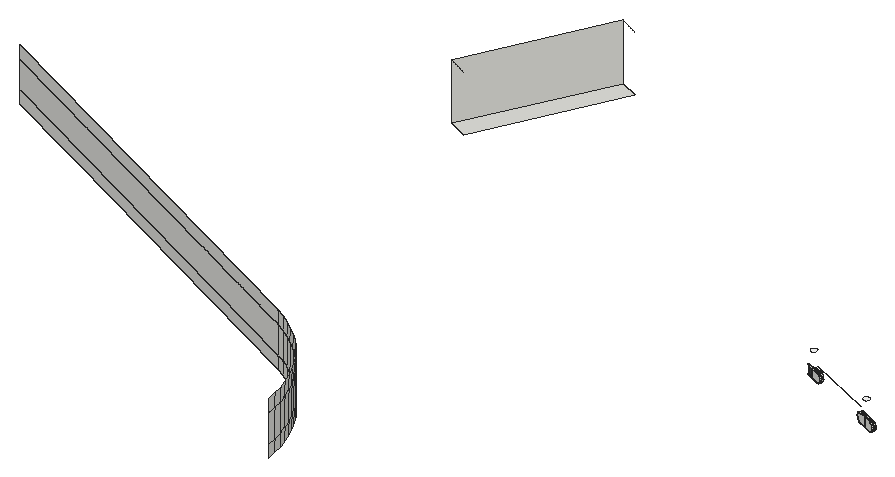
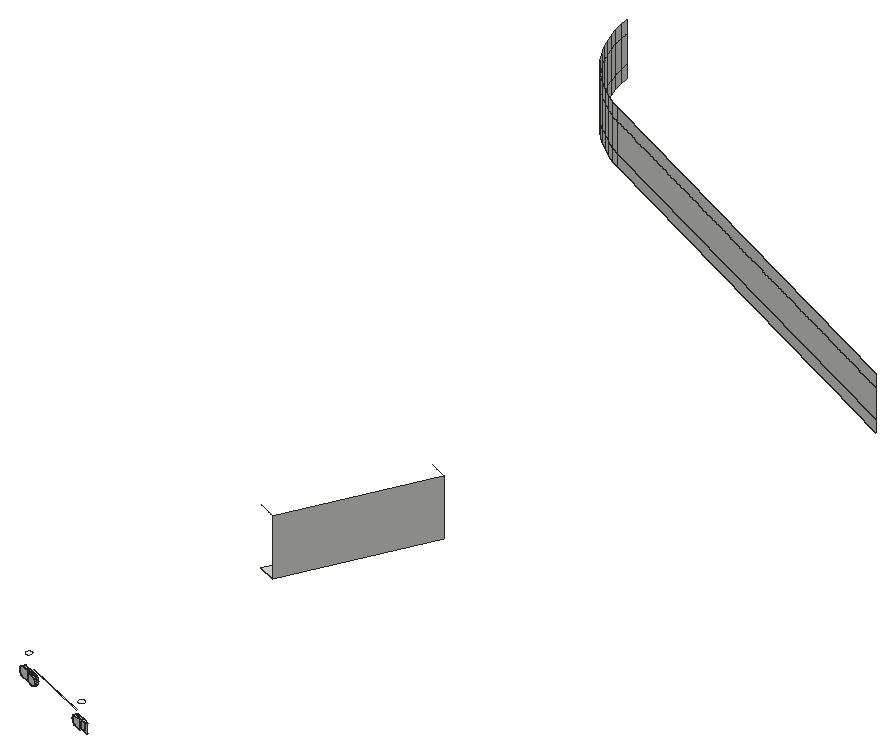
# SketchUp Ruby script. Lengths in inches.
U = 1.inch
M = Sketchup.active_model
def pt(a) = Geom::Point3d.new(a.map { |v| v * U })
def face(e, loops, mat)
  f = e.add_face(loops[0].map { |a| pt(a) })
  loops[1..].each { |l| e.add_face(l.map { |a| pt(a) }).erase! }
  f.material = f.back_material = mat if mat
  f
end
# faces: each face lists its corners as indices into pts; further lists are holes
def faces(e, pts, list, mat = nil) = list.each { |f| face(e, (f[0].is_a?(Array) ? f : [f]).map { |l| l.map { |i| pts[i] } }, mat) }
# xy, xz, yz: faces in a plane at the given z, y or x. An outline is a flat list of corners, or four numbers for a rectangle; further outlines are holes
def ring(l) = l.size == 4 ? [[l[0], l[1]], [l[2], l[1]], [l[2], l[3]], [l[0], l[3]]] : l.each_slice(2).to_a
def flat(e, list, mat, &to3) = list.each { |f| face(e, (f[0].is_a?(Array) ? f : [f]).map { |l| ring(l).map { |u, v| to3.(u, v) } }, mat) }
def xy(e, z, list, mat = nil) = flat(e, list, mat) { |x, y| [x, y, z] }
def xz(e, y, list, mat = nil) = flat(e, list, mat) { |x, z| [x, y, z] }
def yz(e, x, list, mat = nil) = flat(e, list, mat) { |y, z| [x, y, z] }
def lines(e, pts, list) = list.each { |a, b| e.add_line(pt(pts[a]), pt(pts[b])) }
# prism: a flat outline (further loops are holes) pulled along v
def prism(e, loops, v, mat = nil)
  f = face(e, loops, mat); d = Geom::Vector3d.new(v.map { |x| x * U })
  f.pushpull(f.normal.samedirection?(d) ? d.length : -d.length)
end
def box(e, o, s, mat = nil) = prism(e, [[o, [o[0] + s[0], o[1], o[2]], [o[0] + s[0], o[1] + s[1], o[2]], [o[0], o[1] + s[1], o[2]]]], [0, 0, s[2]], mat)
def at(x, y, z, deg = 0) = Geom::Transformation.translation(pt([x, y, z])) * Geom::Transformation.rotation(ORIGIN, Z_AXIS, deg.degrees)
def axes(o, x, y, z) = Geom::Transformation.new([*x, 0, *y, 0, *z, 0, *pt(o).to_a, 1])
def part(name) = M.definitions.add(name)
# library, detail: a bought-in or finely detailed component or shape, given as its bounding box
def library(name, o, s) = part(name).tap { |d| box(d.entities, o, s) }
def detail(e, o, s) = box(e.add_group.entities, o, s)
def put(e, d, t, mat = nil) = e.add_instance(d, t).tap { |i| i.material = mat if mat }
def group(e, t, mat = nil) = e.add_group.tap { |g| g.transformation = t; g.material = mat if mat }.entities
root = M.entities
M.materials.add("Glass_Safety_01").color = [204, 235, 244]
M.materials["Glass_Safety_01"].alpha = 0.1
M.materials.add("[Color_000]").color = [255, 255, 255]
xy(root,351.28,[[958.98,1040.34,957.18,1041.13,957.29,1041.38,958.91,1040.67,959.09,1040.6],[959.17,1040.78,958.99,1040.85,957.36,1041.5625,957.47,1041.82,959.28,1041.03],[957.18,1041.13,955.37,1041.92,955.48,1042.17,957.29,1041.38],[957.36,1041.5625,955.56,1042.35,955.67,1042.6,957.47,1041.82],[939.6,1048.79,937.79,1049.57,937.9,1049.82,939.54,1049.11,939.71,1049.04],
  [939.79,1049.22,939.62,1049.29,937.98,1050.01,938.09,1050.26,939.9,1049.47],[937.79,1049.57,935.99,1050.36,936.1,1050.61,937.9,1049.82]])
xy(root,351.36,[[958.73,1040.75,957.29,1041.38,957.36,1041.5625,958.81,1040.93],[957.29,1041.38,955.84,1042.01,955.92,1042.19,957.36,1041.5625],[939.35,1049.2,937.9,1049.82,937.98,1050.01,939.42,1049.375],[937.9,1049.82,936.46,1050.45,936.54,1050.63,937.98,1050.01]],"Glass_Safety_01")
xy(root,353.33,[[958.73,1040.75,958.81,1040.93,957.36,1041.5625,957.29,1041.38],[957.29,1041.38,957.36,1041.5625,955.92,1042.19,955.84,1042.01],[939.35,1049.2,939.42,1049.375,937.98,1050.01,937.9,1049.82],[937.9,1049.82,937.98,1050.01,936.54,1050.63,936.46,1050.45]],"Glass_Safety_01")
xy(root,353.41,[[958.98,1040.34,959.09,1040.6,958.91,1040.67,957.29,1041.38,957.18,1041.13],[959.17,1040.78,959.28,1041.03,957.47,1041.82,957.36,1041.5625,958.99,1040.85],[957.18,1041.13,957.29,1041.38,955.48,1042.17,955.37,1041.92],[957.36,1041.5625,957.47,1041.82,955.67,1042.6,955.56,1042.35],[939.6,1048.79,939.71,1049.04,939.54,1049.11,937.9,1049.82,937.79,1049.57],
  [939.79,1049.22,939.9,1049.47,938.09,1050.26,937.98,1050.01,939.62,1049.29],[937.79,1049.57,937.9,1049.82,936.1,1050.61,935.99,1050.36]])
xy(root,354.51,[[955.48,1042.17,955.56,1042.35,939.54,1049.11],[955.56,1042.35,939.62,1049.29,939.54,1049.11]],"Glass_Safety_01")
xy(root,357.27,[[957.37,1040.84,957.53,1040.88,957.68,1040.95,957.8,1041.0625,957.89,1041.2,957.94,1041.35,957.95,1041.52,957.92,1041.68,957.85,1041.83,957.74,1041.95,957.6,1042.04,957.44,1042.09,957.28,1042.1,957.12,1042.07,956.97,1041.99,956.85,1041.89,956.76,1041.75,956.71,1041.59,956.7,1041.43,956.73,1041.27,956.8,1041.12,956.91,1041,957.05,1040.91,957.21,1040.85],[937.99,1049.29,938.15,1049.32,938.29,1049.39,938.42,1049.5,938.51,1049.64,938.56,1049.8,938.57,1049.96,938.54,1050.12,938.46,1050.27,938.35,1050.39,938.22,1050.48,938.0625,1050.53,937.9,1050.54,937.74,1050.51,937.59,1050.4375,937.47,1050.33,937.375,1050.19,937.32,1050.03,937.3125,1049.87,937.35,1049.71,937.42,1049.5625,937.53,1049.4375,937.67,1049.35,937.82,1049.3]],"[Color_000]")
xy(root,399.22,[[881.58,1014.85,877.08,1017.03,892.64,1049.08,897.14,1046.9]])
p = [[958.98,1040.34,353.41],[957.18,1041.13,353.41],[957.18,1041.13,351.28],[958.98,1040.34,351.28],[959.23,1040.23,351.32],[959.47,1040.13,351.43],
  [959.67,1040.04,351.59],[959.82,1039.98,351.8125],[959.92,1039.93,352.07],[959.95,1039.92,352.35],[959.92,1039.93,352.62],[959.82,1039.98,352.88],
  [959.67,1040.04,353.1],[959.47,1040.13,353.27],[959.23,1040.23,353.37],[959.34,1040.49,351.32],[959.58,1040.38,351.43],[959.09,1040.6,351.28],
  [958.91,1040.67,351.28],[958.91,1040.67,353.41],[959.09,1040.6,353.41],[959.34,1040.49,353.37],[959.58,1040.38,353.27],[959.78,1040.3,353.1],
  [959.93,1040.23,352.88],[960.03,1040.1875,352.62],[960.06,1040.17,352.35],[960.03,1040.1875,352.07],[959.93,1040.23,351.8125],[959.78,1040.3,351.59],
  [959.17,1040.78,353.41],[958.99,1040.85,353.41],[958.99,1040.85,351.28],[959.17,1040.78,351.28],[959.42,1040.67,351.32],[959.66,1040.57,351.43],
  [959.86,1040.48,351.59],[960.01,1040.41,351.8125],[960.11,1040.37,352.07],[960.14,1040.35,352.35],[960.11,1040.37,352.62],[960.01,1040.41,352.88],
  [959.86,1040.48,353.1],[959.66,1040.57,353.27],[959.42,1040.67,353.37],[957.47,1041.82,353.41],[959.28,1041.03,353.41],[959.53,1040.92,353.37],
  [959.77,1040.82,353.27],[959.97,1040.73,353.1],[960.12,1040.66,352.88],[960.22,1040.62,352.62],[960.25,1040.61,352.35],[960.22,1040.62,352.07],
  [960.12,1040.66,351.8125],[959.97,1040.73,351.59],[959.77,1040.82,351.43],[959.53,1040.92,351.32],[959.28,1041.03,351.28],[957.47,1041.82,351.28],
  [957.29,1041.38,353.41],[957.29,1041.38,351.28],[957.29,1041.38,351.36],[958.73,1040.75,351.36],[958.73,1040.75,353.33],[957.29,1041.38,353.33],
  [957.36,1041.5625,351.28],[957.36,1041.5625,353.41],[957.36,1041.5625,353.33],[958.81,1040.93,353.33],[958.81,1040.93,351.36],[957.36,1041.5625,351.36],
  [955.37,1041.92,353.41],[955.12,1042.03,353.37],[954.88,1042.13,353.27],[954.68,1042.22,353.1],[954.53,1042.28,352.88],[954.43,1042.33,352.62],
  [954.4,1042.34,352.35],[954.43,1042.33,352.07],[954.53,1042.28,351.8125],[954.68,1042.22,351.59],[954.88,1042.13,351.43],[955.12,1042.03,351.32],
  [955.37,1041.92,351.28],[955.48,1042.17,351.28],[955.48,1042.17,353.41],[955.84,1042.01,353.33],[955.84,1042.01,351.36],[955.56,1042.35,353.41],
  [955.56,1042.35,351.28],[955.92,1042.19,351.36],[955.92,1042.19,353.33],[955.67,1042.6,353.41],[955.67,1042.6,351.28],[955.42,1042.71,351.32],
  [955.18,1042.8125,351.43],[954.98,1042.9,351.59],[954.83,1042.97,351.8125],[954.73,1043.01,352.07],[954.69,1043.03,352.35],[954.73,1043.01,352.62],
  [954.83,1042.97,352.88],[954.98,1042.9,353.1],[955.18,1042.8125,353.27],[955.42,1042.71,353.37],[955.23,1042.28,351.32],[954.99,1042.38,351.43],
  [955.23,1042.28,353.37],[954.99,1042.38,353.27],[954.79,1042.47,353.1],[954.64,1042.54,352.88],[954.54,1042.58,352.62],[954.51,1042.59,352.35],
  [954.54,1042.58,352.07],[954.64,1042.54,351.8125],[954.79,1042.47,351.59],[955.31,1042.46,351.32],[955.07,1042.5625,351.43],[954.87,1042.65,351.59],
  [954.72,1042.72,351.8125],[954.62,1042.76,352.07],[954.58,1042.77,352.35],[954.62,1042.76,352.62],[954.72,1042.72,352.88],[954.87,1042.65,353.1],
  [955.07,1042.5625,353.27],[955.31,1042.46,353.37],[939.6,1048.79,353.41],[937.79,1049.57,353.41],[937.79,1049.57,351.28],[939.6,1048.79,351.28],
  [939.85,1048.68,351.32],[940.08,1048.57,351.43],[940.29,1048.49,351.59],[940.44,1048.42,351.8125],[940.54,1048.375,352.07],[940.57,1048.36,352.35],
  [940.54,1048.375,352.62],[940.44,1048.42,352.88],[940.29,1048.49,353.1],[940.08,1048.57,353.27],[939.85,1048.68,353.37],[939.71,1049.04,351.28],
  [939.54,1049.11,351.28],[939.54,1049.11,353.41],[939.71,1049.04,353.41],[939.96,1048.93,353.37],[940.19,1048.83,353.27],[940.4,1048.74,353.1],
  [940.55,1048.67,352.88],[940.65,1048.63,352.62],[940.68,1048.61,352.35],[940.65,1048.63,352.07],[940.55,1048.67,351.8125],[940.4,1048.74,351.59],
  [940.19,1048.83,351.43],[939.96,1048.93,351.32],[939.79,1049.22,353.41],[939.62,1049.29,353.41],[939.62,1049.29,351.28],[939.79,1049.22,351.28],
  [940.04,1049.11,351.32],[940.27,1049.01,351.43],[940.47,1048.92,351.59],[940.63,1048.85,351.8125],[940.73,1048.81,352.07],[940.76,1048.79,352.35],
  [940.73,1048.81,352.62],[940.63,1048.85,352.88],[940.47,1048.92,353.1],[940.27,1049.01,353.27],[940.04,1049.11,353.37],[938.09,1050.26,353.41],
  [939.9,1049.47,353.41],[940.15,1049.36,353.37],[940.38,1049.26,353.27],[940.58,1049.17,353.1],[940.74,1049.1,352.88],[940.84,1049.0625,352.62],
  [940.87,1049.05,352.35],[940.84,1049.0625,352.07],[940.74,1049.1,351.8125],[940.58,1049.17,351.59],[940.38,1049.26,351.43],[940.15,1049.36,351.32],
  [939.9,1049.47,351.28],[938.09,1050.26,351.28],[937.9,1049.82,353.41],[937.9,1049.82,351.28],[937.9,1049.82,351.36],[939.35,1049.2,351.36],
  [939.35,1049.2,353.33],[937.9,1049.82,353.33],[937.98,1050.01,351.28],[937.98,1050.01,353.41],[937.98,1050.01,353.33],[939.42,1049.375,353.33],
  [939.42,1049.375,351.36],[937.98,1050.01,351.36],[936.1,1050.61,351.28],[936.1,1050.61,353.41],[936.46,1050.45,353.33],[936.46,1050.45,351.36],
  [877.08,1017.03,412.84],[892.64,1049.08,412.84],[892.64,1049.08,399.22],[877.08,1017.03,399.22],[945.02,878.89,412.84],[945.02,878.89,415.76],
  [945.42,876.57,415.76],[945.42,876.57,412.84],[944.48,881.18,412.84],[944.48,881.18,415.76],[943.78,883.43,412.84],[943.78,883.43,415.76],
  [942.93,885.63,412.84],[942.93,885.63,415.76],[941.95,887.77,412.84],[941.95,887.77,415.76],[940.83,889.85,412.84],[940.83,889.85,415.76],
  [939.57,891.84,412.84],[939.57,891.84,415.76],[938.1875,893.74,412.84],[938.1875,893.74,415.76],[936.68,895.56,412.84],[936.68,895.56,415.76],
  [935.06,897.27,412.84],[935.06,897.27,415.76],[933.33,898.87,412.84],[933.33,898.87,415.76],[931.5,900.35,412.84],[931.5,900.35,415.76],
  [929.58,901.71,412.84],[929.58,901.71,415.76],[927.57,902.94,412.84],[927.57,902.94,415.76],[925.48,904.04,412.84],[925.48,904.04,415.76],
  [846.42,942.43,412.84],[841.92,944.62,412.84],[824.11,953.26,412.84],[824.11,953.26,415.76],[945.02,878.89,422.51],[945.42,876.57,422.51],
  [944.48,881.18,422.51],[943.78,883.43,422.51],[942.93,885.63,422.51],[941.95,887.77,422.51],[940.83,889.85,422.51],[939.57,891.84,422.51],
  [938.1875,893.74,422.51],[936.68,895.56,422.51],[935.06,897.27,422.51],[933.33,898.87,422.51],[931.5,900.35,422.51],[929.58,901.71,422.51],
  [927.57,902.94,422.51],[925.48,904.04,422.51],[824.11,953.26,422.51],[945.02,878.89,425.53],[945.42,876.57,425.53],[944.48,881.18,425.53],
  [943.78,883.43,425.53],[942.93,885.63,425.53],[941.95,887.77,425.53],[940.83,889.85,425.53],[939.57,891.84,425.53],[938.1875,893.74,425.53],
  [936.68,895.56,425.53],[935.06,897.27,425.53],[933.33,898.87,425.53],[931.5,900.35,425.53],[929.58,901.71,425.53],[927.57,902.94,425.53],
  [925.48,904.04,425.53],[824.11,953.26,425.53],[881.58,1014.85,412.84],[897.14,1046.9,412.84]]
faces(root,p,[[0,1,2,3,4,5,6,7,8,9,10,11,12,13,14],[15,16,5,4],[17,18,19,20,21,22,23,24,25,26,27,28,29,16,15],[17,15,4,3],[30,31,32,33,34,35,36,37,38,39,40,41,42,43,44],[45,46,47,48,49,50,51,52,53,54,55,56,57,58,59],[35,34,57,56],[60,19,18,61,62,63,64,65],
  [34,33,58,57],[66,32,31,67,68,69,70,71],[1,72,73,74,75,76,77,78,79,80,81,82,83,84,2],[62,61,2,1,60,65],[61,85,86,60,65,87,88,62],[67,89,90,66,71,91,92,68],[66,71,68,67,45,59],[93,45,59,94,95,96,97,98,99,100,101,102,103,104,105],
  [106,85,84,83],[107,106,83,82],[90,117,95,94],[117,118,96,95],[128,129,130,131,132,133,134,135,136,137,138,139,140,141,142],[143,144,145,146,147,148,149,150,151,152,153,154,155,156,157],[157,156,133,132],[143,157,132,131],
  [158,159,160,161,162,163,164,165,166,167,168,169,170,171,172],[173,174,175,176,177,178,179,180,181,182,183,184,185,186,187],[163,162,185,184],[188,145,144,189,190,191,192,193],[162,161,186,185],[194,160,159,195,196,197,198,199],[190,189,130,129,188,193],[189,200,201,188,193,202,203,190],
  [194,199,196,195,173,187],[16,29,6,5],[36,35,56,55],[116,107,82,81],[118,119,97,96],[156,155,134,133],[164,163,184,183],[29,28,7,6],
  [37,36,55,54],[115,116,81,80],[119,120,98,97],[155,154,135,134],[165,164,183,182],[28,27,8,7],[38,37,54,53],[114,115,80,79],
  [120,121,99,98],[154,153,136,135],[166,165,182,181],[27,26,9,8],[39,38,53,52],[113,114,79,78],[121,122,100,99],[153,152,137,136],
  [167,166,181,180],[26,25,10,9],[40,39,52,51],[112,113,78,77],[122,123,101,100],[152,151,138,137],[168,167,180,179],[25,24,11,10],
  [41,40,51,50],[111,112,77,76],[123,124,102,101],[151,150,139,138],[169,168,179,178],[24,23,12,11],[42,41,50,49],[110,111,76,75],
  [124,125,103,102],[150,149,140,139],[170,169,178,177],[23,22,13,12],[43,42,49,48],[109,110,75,74],[125,126,104,103],[149,148,141,140],
  [171,170,177,176],[22,21,14,13],[44,43,48,47],[108,109,74,73],[126,127,105,104],[148,147,142,141],[172,171,176,175],[21,20,0,14],
  [30,44,47,46],[86,108,73,72],[127,89,93,105],[147,146,128,142],[158,172,175,174],[204,205,206,207],[208,209,210,211],[212,213,209,208],
  [214,215,213,212],[216,217,215,214],[218,219,217,216],[220,221,219,218],[222,223,221,220],[224,225,223,222],[226,227,225,224],[228,229,227,226],
  [230,231,229,228],[232,233,231,230],[234,235,233,232],[236,237,235,234],[238,239,237,236],[238,240,241,242,243,239],[210,209,244,245],[209,213,246,244],
  [213,215,247,246],[215,217,248,247],[217,219,249,248],[219,221,250,249],[221,223,251,250],[223,225,252,251],[225,227,253,252],[227,229,254,253],
  [229,231,255,254],[231,233,256,255],[233,235,257,256],[235,237,258,257],[237,239,259,258],[239,243,260,259],[245,244,261,262],[244,246,263,261],
  [246,247,264,263],[247,248,265,264],[248,249,266,265],[249,250,267,266],[250,251,268,267],[251,252,269,268],[252,253,270,269],[253,254,271,270],
  [254,255,272,271],[255,256,273,272],[256,257,274,273],[257,258,275,274],[258,259,276,275],[259,260,277,276]])
faces(root,p,[[85,86,108,109,110,111,112,113,114,115,116,107,106],[89,90,117,118,119,120,121,122,123,124,125,126,127],[65,64,63,62],[64,63,70,69],[69,68,71,70],[87,65,62,88],[65,68,71,62],[68,92,91,71],
  [92,91,88,87],[193,192,191,190],[192,191,198,197],[197,196,199,198],[202,193,190,203],[193,196,199,190]],"Glass_Safety_01")
lines(root,p,[[204,278],[205,279]])
